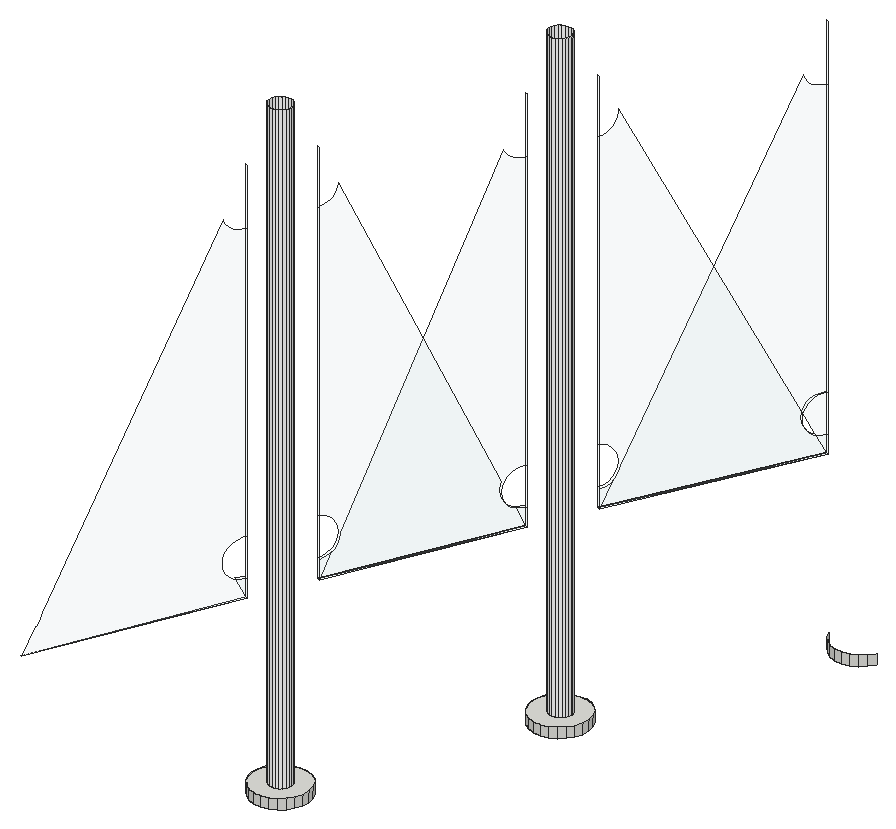
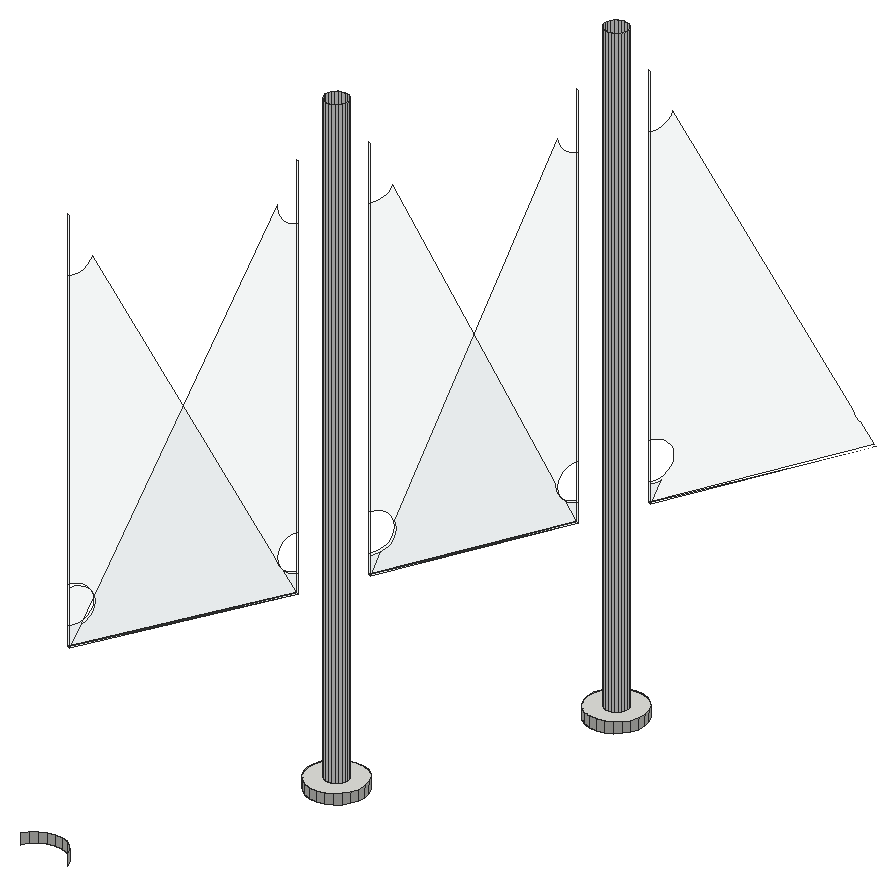
# SketchUp Ruby script. Lengths in inches.
U = 1.inch
M = Sketchup.active_model
def pt(a) = Geom::Point3d.new(a.map { |v| v * U })
def face(e, loops, mat)
  f = e.add_face(loops[0].map { |a| pt(a) })
  loops[1..].each { |l| e.add_face(l.map { |a| pt(a) }).erase! }
  f.material = f.back_material = mat if mat
  f
end
# faces: each face lists its corners as indices into pts; further lists are holes
def faces(e, pts, list, mat = nil) = list.each { |f| face(e, (f[0].is_a?(Array) ? f : [f]).map { |l| l.map { |i| pts[i] } }, mat) }
# xy, xz, yz: faces in a plane at the given z, y or x. An outline is a flat list of corners, or four numbers for a rectangle; further outlines are holes
def ring(l) = l.size == 4 ? [[l[0], l[1]], [l[2], l[1]], [l[2], l[3]], [l[0], l[3]]] : l.each_slice(2).to_a
def flat(e, list, mat, &to3) = list.each { |f| face(e, (f[0].is_a?(Array) ? f : [f]).map { |l| ring(l).map { |u, v| to3.(u, v) } }, mat) }
def xy(e, z, list, mat = nil) = flat(e, list, mat) { |x, y| [x, y, z] }
def xz(e, y, list, mat = nil) = flat(e, list, mat) { |x, z| [x, y, z] }
def yz(e, x, list, mat = nil) = flat(e, list, mat) { |y, z| [x, y, z] }
def lines(e, pts, list) = list.each { |a, b| e.add_line(pt(pts[a]), pt(pts[b])) }
# prism: a flat outline (further loops are holes) pulled along v
def prism(e, loops, v, mat = nil)
  f = face(e, loops, mat); d = Geom::Vector3d.new(v.map { |x| x * U })
  f.pushpull(f.normal.samedirection?(d) ? d.length : -d.length)
end
def box(e, o, s, mat = nil) = prism(e, [[o, [o[0] + s[0], o[1], o[2]], [o[0] + s[0], o[1] + s[1], o[2]], [o[0], o[1] + s[1], o[2]]]], [0, 0, s[2]], mat)
def at(x, y, z, deg = 0) = Geom::Transformation.translation(pt([x, y, z])) * Geom::Transformation.rotation(ORIGIN, Z_AXIS, deg.degrees)
def axes(o, x, y, z) = Geom::Transformation.new([*x, 0, *y, 0, *z, 0, *pt(o).to_a, 1])
def part(name) = M.definitions.add(name)
# library, detail: a bought-in or finely detailed component or shape, given as its bounding box
def library(name, o, s) = part(name).tap { |d| box(d.entities, o, s) }
def detail(e, o, s) = box(e.add_group.entities, o, s)
def put(e, d, t, mat = nil) = e.add_instance(d, t).tap { |i| i.material = mat if mat }
def group(e, t, mat = nil) = e.add_group.tap { |g| g.transformation = t; g.material = mat if mat }.entities
root = M.entities
M.materials.add("Glass_Safety_01").color = [204, 235, 244]
M.materials["Glass_Safety_01"].alpha = 0.1
M.materials.add("[Color_000]").color = [255, 255, 255]
xy(root,321.27,[[[871.11,598.11,871.51,598.19,871.88,598.38,872.1875,598.65,872.42,598.99,872.55,599.38,872.57,599.79,872.49,600.2,872.3,600.5625,872.03,600.87,871.6875,601.1,871.625,601.12,871.3,601.23,870.89,601.25,870.48,601.17,870.12,600.99,869.81,600.71,869.58,600.37,869.45,599.98,869.43,599.57,869.51,599.17,869.69,598.8,869.97,598.49,870.3125,598.26,870.37,598.24,870.7,598.13],[871.04,599.05,870.88,599.0625,870.75,599.11,870.72,599.11,870.59,599.2,870.48,599.33,870.4,599.47,870.37,599.64,870.38,599.8,870.43,599.96,870.52,600.09,870.65,600.2,870.79,600.28,870.95,600.31,871.12,600.3,871.25,600.26,871.27,600.25,871.41,600.16,871.52,600.03,871.59,599.89,871.625,599.73,871.62,599.5625,871.57,599.41,871.47,599.27,871.35,599.16,871.2,599.09]],[870.37,598.24,870.75,599.11,870.72,599.11,870.59,599.2,870.48,599.33,870.4,599.47,870.37,599.64,870.38,599.8,870.43,599.96,870.52,600.09,870.65,600.2,870.79,600.28,870.95,600.31,871.12,600.3,871.25,600.26,871.625,601.12,871.3,601.23,870.89,601.25,870.48,601.17,870.12,600.99,869.81,600.71,869.58,600.37,869.45,599.98,869.43,599.57,869.51,599.17,869.69,598.8,869.97,598.49,870.3125,598.26],[870.72,599.11,870.75,599.11,871.25,600.26,871.12,600.3,870.95,600.31,870.79,600.28,870.65,600.2,870.52,600.09,870.43,599.96,870.38,599.8,870.37,599.64,870.4,599.47,870.48,599.33,870.59,599.2],[[876.92,611.23,877.32,611.31,877.6875,611.5,877.99,611.77,878.22,612.12,878.35,612.51,878.375,612.92,878.29,613.32,878.11,613.6875,877.83,613.99,877.49,614.22,877.35,614.27,877.1,614.35,876.69,614.375,876.29,614.29,875.92,614.11,875.61,613.83,875.39,613.49,875.26,613.1,875.23,612.69,875.32,612.29,875.5,611.92,875.77,611.61,876.1,611.4,876.12,611.39,876.51,611.26],[876.85,612.17,876.68,612.18,876.53,612.24,876.48,612.27,876.39,612.33,876.28,612.45,876.21,612.6,876.18,612.76,876.19,612.92,876.24,613.08,876.33,613.22,876.45,613.32,876.6,613.4,876.76,613.43,876.92,613.42,876.98,613.4,877.08,613.37,877.22,613.28,877.33,613.16,877.4,613.01,877.43,612.85,877.42,612.68,877.37,612.53,877.28,612.39,877.16,612.28,877.01,612.21]],[876.1,611.4,876.48,612.27,876.39,612.33,876.28,612.45,876.21,612.6,876.18,612.76,876.19,612.92,876.24,613.08,876.33,613.22,876.45,613.32,876.6,613.4,876.76,613.43,876.92,613.42,876.98,613.4,877.35,614.27,877.1,614.35,876.69,614.375,876.29,614.29,875.92,614.11,875.61,613.83,875.39,613.49,875.26,613.1,875.23,612.69,875.32,612.29,875.5,611.92,875.77,611.61],
  [876.48,612.27,876.98,613.4,876.92,613.42,876.76,613.43,876.6,613.4,876.45,613.32,876.33,613.22,876.24,613.08,876.19,612.92,876.18,612.76,876.21,612.6,876.28,612.45,876.39,612.33]])
xy(root,321.27,[[871.04,599.05,871.2,599.09,871.35,599.16,871.47,599.27,871.57,599.41,871.62,599.5625,871.625,599.73,871.59,599.89,871.52,600.03,871.41,600.16,871.27,600.25,871.25,600.26,870.75,599.11,870.88,599.0625],[876.85,612.17,877.01,612.21,877.16,612.28,877.28,612.39,877.37,612.53,877.42,612.68,877.43,612.85,877.4,613.01,877.33,613.16,877.22,613.28,877.08,613.37,876.98,613.4,876.48,612.27,876.53,612.24,876.68,612.18]],"[Color_000]")
xy(root,321.86,[[871.11,598.11,871.51,598.19,871.88,598.38,872.1875,598.65,872.42,598.99,872.55,599.38,872.57,599.79,872.49,600.2,872.3,600.5625,872.03,600.87,871.6875,601.1,871.3,601.23,870.89,601.25,870.48,601.17,870.12,600.99,869.81,600.71,869.58,600.37,869.45,599.98,869.43,599.57,869.51,599.17,869.69,598.8,869.97,598.49,870.3125,598.26,870.7,598.13],[876.92,611.23,877.32,611.31,877.6875,611.5,877.99,611.77,878.22,612.12,878.35,612.51,878.375,612.92,878.29,613.32,878.11,613.6875,877.83,613.99,877.49,614.22,877.1,614.35,876.69,614.375,876.29,614.29,875.92,614.11,875.61,613.83,875.39,613.49,875.26,613.1,875.23,612.69,875.32,612.29,875.5,611.92,875.77,611.61,876.12,611.39,876.51,611.26]])
xy(root,331.9,[[865.59,587.5,870.22,598.15,870.4,598.07],[871.89,601.44,871.71,601.52,876.21,611.21],[871.71,601.52,876.03,611.29,876.21,611.21],[877.73,614.54,877.56,614.625,882.68,625.01],[877.56,614.625,882.5,625.09,882.68,625.01]],"Glass_Safety_01")
p = [[870.3125,598.26,321.27],[870.37,598.24,321.27],[870.7,598.13,321.27],[870.7,598.13,321.86],[870.3125,598.26,321.86],[871.11,598.11,321.27],
  [871.11,598.11,321.86],[871.51,598.19,321.27],[871.51,598.19,321.86],[871.88,598.38,321.27],[871.88,598.38,321.86],[869.97,598.49,321.27],
  [869.97,598.49,321.86],[872.1875,598.65,321.27],[872.1875,598.65,321.86],[869.69,598.8,321.27],[869.69,598.8,321.86],[872.42,598.99,321.27],
  [872.42,598.99,321.86],[869.51,599.17,321.27],[869.51,599.17,321.86],[872.55,599.38,321.27],[872.55,599.38,321.86],[870.59,599.2,321.27],
  [870.72,599.11,321.27],[870.72,599.11,357.27],[870.59,599.2,357.27],[870.75,599.11,321.27],[870.88,599.0625,321.27],[870.88,599.0625,357.27],
  [871.04,599.05,321.27],[871.04,599.05,357.27],[871.2,599.09,321.27],[871.2,599.09,357.27],[871.35,599.16,321.27],[871.35,599.16,357.27],
  [869.43,599.57,321.27],[869.43,599.57,321.86],[870.48,599.33,321.27],[870.48,599.33,357.27],[871.47,599.27,321.27],[871.47,599.27,357.27],
  [870.4,599.47,321.27],[870.4,599.47,357.27],[871.57,599.41,321.27],[871.57,599.41,357.27],[871.62,599.5625,321.27],[871.62,599.5625,357.27],
  [872.57,599.79,321.27],[872.57,599.79,321.86],[870.37,599.64,321.27],[870.37,599.64,357.27],[869.45,599.98,321.27],[869.45,599.98,321.86],
  [870.38,599.8,321.27],[870.38,599.8,357.27],[871.625,599.73,321.27],[871.625,599.73,357.27],[871.59,599.89,321.27],[871.59,599.89,357.27],
  [870.43,599.96,321.27],[870.43,599.96,357.27],[872.49,600.2,321.27],[872.49,600.2,321.86],[871.52,600.03,321.27],[871.52,600.03,357.27],
  [869.58,600.37,321.27],[869.58,600.37,321.86],[870.52,600.09,321.27],[870.52,600.09,357.27],[871.41,600.16,321.27],[871.41,600.16,357.27],
  [870.65,600.2,321.27],[870.65,600.2,357.27],[870.79,600.28,321.27],[870.79,600.28,357.27],[871.27,600.25,321.27],[871.25,600.26,321.27],
  [871.12,600.3,321.27],[871.12,600.3,357.27],[871.27,600.25,357.27],[872.3,600.5625,321.27],[872.3,600.5625,321.86],[870.95,600.31,321.27],
  [870.95,600.31,357.27],[869.81,600.71,321.27],[869.81,600.71,321.86],[872.03,600.87,321.27],[872.03,600.87,321.86],[870.12,600.99,321.27],
  [870.12,600.99,321.86],[871.6875,601.1,321.27],[871.6875,601.1,321.86],[870.48,601.17,321.27],[870.48,601.17,321.86],[871.625,601.12,321.27],
  [871.3,601.23,321.27],[871.3,601.23,321.86],[870.89,601.25,321.27],[870.89,601.25,321.86],[876.51,611.26,321.27],[876.92,611.23,321.27],
  [876.92,611.23,321.86],[876.51,611.26,321.86],[877.32,611.31,321.27],[877.32,611.31,321.86],[876.12,611.39,321.27],[876.12,611.39,321.86],
  [877.6875,611.5,321.27],[877.6875,611.5,321.86],[875.77,611.61,321.27],[876.1,611.4,321.27],[875.77,611.61,321.86],[877.99,611.77,321.27],
  [877.99,611.77,321.86],[875.5,611.92,321.27],[875.5,611.92,321.86],[878.22,612.12,321.27],[878.22,612.12,321.86],[875.32,612.29,321.27],
  [875.32,612.29,321.86],[878.35,612.51,321.27],[878.35,612.51,321.86],[876.39,612.33,321.27],[876.48,612.27,321.27],[876.53,612.24,321.27],
  [876.53,612.24,357.27],[876.39,612.33,357.27],[876.68,612.18,321.27],[876.68,612.18,357.27],[876.85,612.17,321.27],[876.85,612.17,357.27],
  [877.01,612.21,321.27],[877.01,612.21,357.27],[877.16,612.28,321.27],[877.16,612.28,357.27],[875.23,612.69,321.27],[875.23,612.69,321.86],
  [876.28,612.45,321.27],[876.28,612.45,357.27],[877.28,612.39,321.27],[877.28,612.39,357.27],[876.21,612.6,321.27],[876.21,612.6,357.27],
  [877.37,612.53,321.27],[877.37,612.53,357.27],[877.42,612.68,321.27],[877.42,612.68,357.27],[878.375,612.92,321.27],[878.375,612.92,321.86],
  [876.18,612.76,321.27],[876.18,612.76,357.27],[875.26,613.1,321.27],[875.26,613.1,321.86],[877.43,612.85,321.27],[877.43,612.85,357.27],
  [876.19,612.92,321.27],[876.19,612.92,357.27],[877.4,613.01,321.27],[877.4,613.01,357.27],[876.24,613.08,321.27],[876.24,613.08,357.27],
  [878.29,613.32,321.27],[878.29,613.32,321.86],[877.33,613.16,321.27],[877.33,613.16,357.27],[875.39,613.49,321.27],[875.39,613.49,321.86],
  [876.33,613.22,321.27],[876.33,613.22,357.27],[876.45,613.32,321.27],[876.45,613.32,357.27],[877.22,613.28,321.27],[877.22,613.28,357.27],
  [876.6,613.4,321.27],[876.6,613.4,357.27],[877.08,613.37,321.27],[877.08,613.37,357.27],[878.11,613.6875,321.27],[878.11,613.6875,321.86],
  [876.76,613.43,321.27],[876.76,613.43,357.27],[876.92,613.42,321.27],[876.92,613.42,357.27],[876.98,613.4,321.27],[875.61,613.83,321.27],
  [875.61,613.83,321.86],[877.83,613.99,321.27],[877.83,613.99,321.86],[875.92,614.11,321.27],[875.92,614.11,321.86],[877.49,614.22,321.27],
  [877.49,614.22,321.86],[876.29,614.29,321.27],[876.29,614.29,321.86],[877.35,614.27,321.27],[877.1,614.35,321.27],[877.1,614.35,321.86],
  [876.69,614.375,321.27],[876.69,614.375,321.86],[883.03,625.05,321.27],[883.4375,625.03,321.27],[883.4375,625.03,321.86],[883.03,625.05,321.86],
  [883.84,625.11,321.27],[883.84,625.11,321.86],[882.64,625.18,321.27],[882.64,625.18,321.86],[884.21,625.3,321.27],[884.21,625.3,321.86],
  [882.29,625.41,321.27],[882.29,625.41,321.86],[884.51,625.57,321.27],[884.51,625.57,321.86],[882.02,625.72,321.27],[882.23,625.48,321.27],
  [882.02,625.72,321.86],[884.74,625.91,321.27],[884.74,625.91,321.86],[881.84,626.09,321.27],[881.84,626.09,321.86],[870.4,598.07,335.125],
  [870.4,598.07,351.28],[870.3,597.84,351.28],[870.19,597.58,351.32],[870.09,597.35,351.43],[870,597.15,351.59],[869.94,596.99,351.81],
  [869.9,596.91,352.04],[866.18,588.38,333.93],[866.18,588.36,333.79],[866.13,588.26,333.53],[866.07,588.11,333.3125],[866.05,588.07,333.28],
  [865.77,587.42,331.9],[870.4,598.07,331.9],[870.4,598.07,333],[870.3,597.84,333],[870.19,597.58,333.04],[870.09,597.35,333.14],
  [870,597.15,333.3125],[869.94,596.99,333.53],[869.89,596.9,333.79],[869.88,596.86,334.0625],[869.89,596.9,334.34],[869.94,596.99,334.59],
  [870,597.15,334.8125],[870.09,597.35,334.98],[870.19,597.58,335.09],[870.3,597.84,335.125],[870.22,598.15,331.9],[869.98,597.6,333.07],
  [870.01,597.66,333.04],[870.12,597.92,333],[870.22,598.15,333],[870.22,598.15,335.125],[870.22,598.15,351.28],[870.22,598.15,353.41],
  [870.22,598.15,354.51],[870.4,598.07,354.51],[870.4,598.07,353.41],[871.71,601.52,331.9],[871.89,601.44,331.9],[871.89,601.44,333],
  [871.89,601.44,335.125],[871.89,601.44,351.28],[871.89,601.44,353.41],[871.89,601.44,354.51],[871.71,601.52,354.51],[871.71,601.52,353.41],
  [871.71,601.52,351.28],[871.71,601.52,335.125],[871.71,601.52,333],[872.14,602.01,333.21],[872.1,601.93,333.14],[872,601.69,333.04],
  [875.71,610.09,351.91],[872.3125,602.41,334.13],[872.32,602.41,334.0625],[872.3,602.38,333.79],[872.26,602.28,333.53],[872.1875,602.13,333.3125],
  [876.21,611.21,331.9],[876.21,611.21,333],[876.1,610.96,333],[875.99,610.71,333.04],[875.88,610.48,333.14],[875.79,610.28,333.3125],
  [875.72,610.12,333.53],[875.68,610.02,333.79],[875.67,609.99,334.0625],[875.68,610.02,334.34],[875.72,610.12,334.59],[875.79,610.28,334.8125],
  [875.88,610.48,334.98],[875.99,610.71,335.09],[876.1,610.96,335.125],[876.21,611.21,335.125],[876.21,611.21,351.28],[876.1,610.96,351.28],
  [875.99,610.71,351.32],[875.88,610.48,351.43],[875.79,610.28,351.59],[875.72,610.12,351.8125],[871.82,601.77,351.32],[871.92,602.01,351.43],
  [872.01,602.21,351.59],[872.08,602.36,351.81],[872.12,602.46,352.07],[872.13,602.49,352.28],[875.53,610.17,334.5],[875.5,610.1,334.34],
  [875.49,610.07,334.0625],[875.5,610.1,333.79],[875.54,610.2,333.53],[875.61,610.36,333.3125],[875.7,610.56,333.14],[875.81,610.79,333.04],
  [875.81,610.8,333.03],[876.03,611.29,331.9],[871.82,601.77,333.04],[871.92,602.01,333.14],[872.01,602.21,333.3125],[872.08,602.36,333.53],
  [872.12,602.46,333.79],[872.14,602.49,334.0625],[872.12,602.46,334.34],[872.08,602.36,334.59],[872.01,602.21,334.8125],[871.92,602.01,334.98],
  [871.82,601.77,335.09],[875.92,611.04,333],[876.03,611.29,333],[876.03,611.29,335.125],[876.03,611.29,351.28],[876.03,611.29,353.41],
  [876.03,611.29,354.51],[876.21,611.21,354.51],[876.21,611.21,353.41],[877.56,614.625,331.9],[877.73,614.54,331.9],[877.73,614.54,333],
  [877.73,614.54,335.125],[877.73,614.54,351.28],[877.73,614.54,353.41],[877.73,614.54,354.51],[877.56,614.625,354.51],[877.56,614.625,353.41],
  [877.56,614.625,351.28],[877.56,614.625,335.125],[877.56,614.625,333],[878.04,615.18,333.28],[877.96,615.02,333.14],[877.85,614.79,333.04],
  [882.68,625.01,335.125],[882.68,625.01,351.28],[882.57,624.78,351.28],[882.45,624.53,351.32],[882.35,624.3,351.43],[882.25,624.1,351.59],
  [882.18,623.95,351.8125],[882.14,623.86,352.04],[878.18,615.49,333.94],[878.17,615.47,333.79],[878.13,615.37,333.53],[878.05,615.22,333.3125],
  [882.68,625.01,331.9],[882.68,625.01,333],[882.57,624.78,333],[882.45,624.53,333.04],[882.35,624.3,333.14],[882.25,624.1,333.3125],
  [882.18,623.95,333.53],[882.13,623.85,333.79],[882.12,623.82,334.0625],[882.13,623.85,334.34],[882.18,623.95,334.59],[882.25,624.1,334.8125],
  [882.35,624.3,334.98],[882.45,624.53,335.09],[882.57,624.78,335.125],[878,615.57,352.47],[881.96,623.95,334.37],[881.96,623.93,334.34],
  [881.94,623.9,334.0625],[881.96,623.93,333.79],[882,624.03,333.53],[882.07,624.18,333.3125],[882.17,624.38,333.14],[882.25,624.55,333.0625],
  [882.5,625.09,331.9],[877.67,614.875,333.04],[877.78,615.11,333.14],[877.875,615.3,333.3125],[877.95,615.46,333.53],[877.99,615.55,333.79],
  [878.01,615.59,334.0625],[877.99,615.55,334.34],[877.95,615.46,334.59],[877.875,615.3,334.8125],[877.78,615.11,334.98],[877.67,614.875,335.09],
  [877.67,614.875,351.32],[877.78,615.11,351.43],[877.875,615.3,351.59],[877.95,615.46,351.8125],[877.99,615.55,352.07],[878.01,615.59,352.35],
  [882,624.03,334.59],[882.07,624.18,334.8125],[882.17,624.38,334.98],[882.28,624.61,335.09],[882.39,624.86,335.125],[882.5,625.09,335.125],
  [882.5,625.09,333],[882.5,625.09,351.28],[882.5,625.09,353.41],[882.5,625.09,354.51],[882.68,625.01,354.51],[882.68,625.01,353.41]]
faces(root,p,[[0,1,2,3,4],[2,5,6,3],[5,7,8,6],[7,9,10,8],[11,0,4,12],[9,13,14,10],[15,11,12,16],[13,17,18,14],
  [19,15,16,20],[17,21,22,18],[36,19,20,37],[21,48,49,22],[52,36,37,53],[48,62,63,49],[66,52,53,67],[62,81,82,63],
  [85,66,67,86],[81,87,88,82],[89,85,86,90],[87,91,92,88],[93,89,90,94],[91,95,96,97,92],[98,93,94,99],[96,98,99,97],
  [100,101,102,103],[101,104,105,102],[106,100,103,107],[104,108,109,105],[110,111,106,107,112],[108,113,114,109],[115,110,112,116],[113,117,118,114],
  [119,115,116,120],[117,121,122,118],[136,119,120,137],[121,148,149,122],[152,136,137,153],[148,162,163,149],[166,152,153,167],[162,178,179,163],
  [185,166,167,186],[178,187,188,179],[189,185,186,190],[187,191,192,188],[193,189,190,194],[191,195,196,197,192],[198,193,194,199],[196,198,199,197],
  [200,201,202,203],[201,204,205,202],[206,200,203,207],[204,208,209,205],[210,206,207,211],[208,212,213,209],[214,215,210,211,216],[212,217,218,213],
  [219,214,216,220]])
faces(root,p,[[23,24,25,26],[24,27,28,29,25],[28,30,31,29],[30,32,33,31],[32,34,35,33],[38,23,26,39],[34,40,41,35],[42,38,39,43],
  [40,44,45,41],[44,46,47,45],[50,42,43,51],[54,50,51,55],[46,56,57,47],[56,58,59,57],[60,54,55,61],[58,64,65,59],
  [68,60,61,69],[64,70,71,65],[72,68,69,73],[74,72,73,75],[76,77,78,79,80],[70,76,80,71],[83,74,75,84],[78,83,84,79],
  [123,124,125,126,127],[125,128,129,126],[128,130,131,129],[130,132,133,131],[132,134,135,133],[138,123,127,139],[134,140,141,135],[142,138,139,143],
  [140,144,145,141],[144,146,147,145],[150,142,143,151],[146,154,155,147],[156,150,151,157],[154,158,159,155],[160,156,157,161],[158,164,165,159],
  [168,160,161,169],[170,168,169,171],[164,172,173,165],[174,170,171,175],[172,176,177,173],[180,174,175,181],[182,180,181,183],[176,184,182,183,177]],"[Color_000]")
faces(root,p,[[221,222,223,224,225,226,227,228,229,230,231,232,233,234,235,236,237,238,239,240,241,242,243,244,245,246,247,248,249],[250,251,252,253,254],[235,250,254,255,256,257,258,259,260,222,221,236],[261,262,263,264,265,266,267,268,269,270,271,272],[262,273,274,275,263],[276,277,278,279,280,281,273,262,282,283,284,285,286,287,288,289,290,291,292,293,294,295,296,297,298,299,300,301,302,303],[271,270,304,305,306,307,308,309,310,311,312,313,314,315,316,317,318,319,261,272,320,321,322,323,324,325,326,327,328,329,330],[319,318,331,332],
  [282,319,332,333,334,335,336,337,338,298,297,283],[339,340,341,342,343,344,345,346,347,348,349,350],[340,351,352,353,341],[354,355,356,357,358,359,360,361,362,363,364,365,351,340,366,367,368,369,370,371,372,373,374,375,376,377,378,379,380],[381,382,383,384,385,386,387,388,389,390,339,350,391,392,393,394,395,396,397,398,399,400,401,349,348,402,403,404,405,406,407],[389,382,408,409,410,411,412,413,414,390],[366,390,414,413,415,416,417,418,419,355,354,367]],"Glass_Safety_01")
